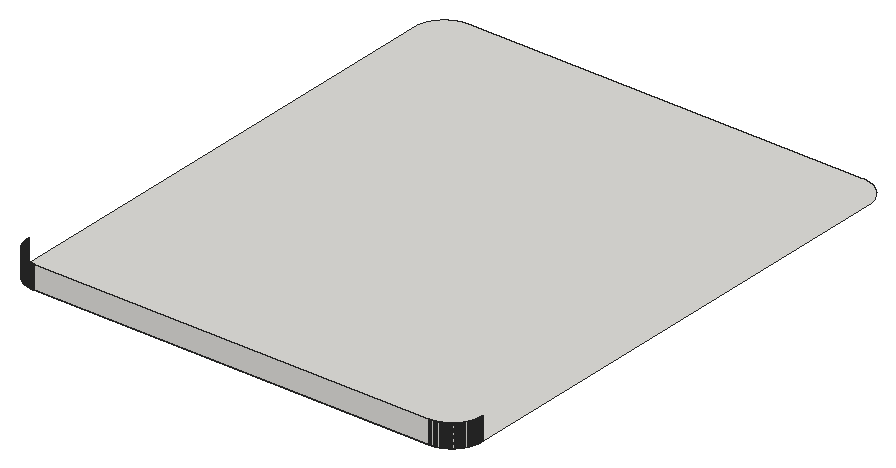
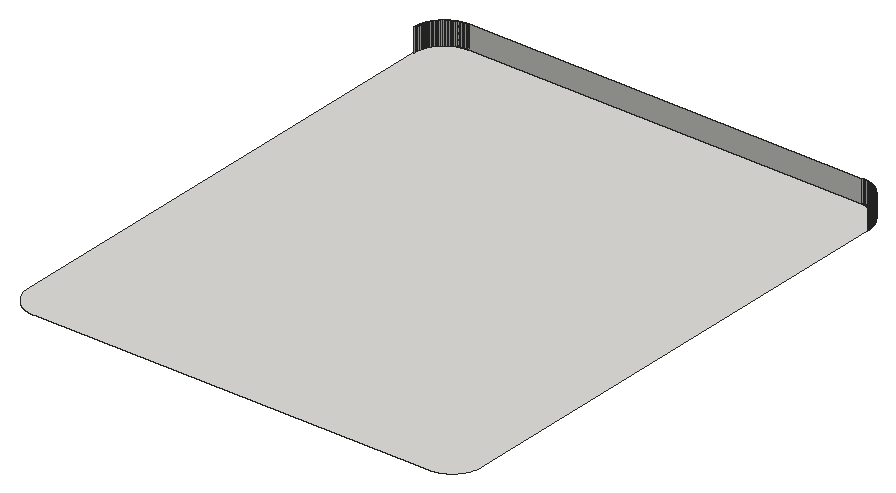
# SketchUp Ruby script. Lengths in inches.
U = 1.inch
M = Sketchup.active_model
def pt(a) = Geom::Point3d.new(a.map { |v| v * U })
def face(e, loops, mat)
  f = e.add_face(loops[0].map { |a| pt(a) })
  loops[1..].each { |l| e.add_face(l.map { |a| pt(a) }).erase! }
  f.material = f.back_material = mat if mat
  f
end
# faces: each face lists its corners as indices into pts; further lists are holes
def faces(e, pts, list, mat = nil) = list.each { |f| face(e, (f[0].is_a?(Array) ? f : [f]).map { |l| l.map { |i| pts[i] } }, mat) }
# xy, xz, yz: faces in a plane at the given z, y or x. An outline is a flat list of corners, or four numbers for a rectangle; further outlines are holes
def ring(l) = l.size == 4 ? [[l[0], l[1]], [l[2], l[1]], [l[2], l[3]], [l[0], l[3]]] : l.each_slice(2).to_a
def flat(e, list, mat, &to3) = list.each { |f| face(e, (f[0].is_a?(Array) ? f : [f]).map { |l| ring(l).map { |u, v| to3.(u, v) } }, mat) }
def xy(e, z, list, mat = nil) = flat(e, list, mat) { |x, y| [x, y, z] }
def xz(e, y, list, mat = nil) = flat(e, list, mat) { |x, z| [x, y, z] }
def yz(e, x, list, mat = nil) = flat(e, list, mat) { |y, z| [x, y, z] }
def lines(e, pts, list) = list.each { |a, b| e.add_line(pt(pts[a]), pt(pts[b])) }
# prism: a flat outline (further loops are holes) pulled along v
def prism(e, loops, v, mat = nil)
  f = face(e, loops, mat); d = Geom::Vector3d.new(v.map { |x| x * U })
  f.pushpull(f.normal.samedirection?(d) ? d.length : -d.length)
end
def box(e, o, s, mat = nil) = prism(e, [[o, [o[0] + s[0], o[1], o[2]], [o[0] + s[0], o[1] + s[1], o[2]], [o[0], o[1] + s[1], o[2]]]], [0, 0, s[2]], mat)
def at(x, y, z, deg = 0) = Geom::Transformation.translation(pt([x, y, z])) * Geom::Transformation.rotation(ORIGIN, Z_AXIS, deg.degrees)
def axes(o, x, y, z) = Geom::Transformation.new([*x, 0, *y, 0, *z, 0, *pt(o).to_a, 1])
def part(name) = M.definitions.add(name)
# library, detail: a bought-in or finely detailed component or shape, given as its bounding box
def library(name, o, s) = part(name).tap { |d| box(d.entities, o, s) }
def detail(e, o, s) = box(e.add_group.entities, o, s)
def put(e, d, t, mat = nil) = e.add_instance(d, t).tap { |i| i.material = mat if mat }
def group(e, t, mat = nil) = e.add_group.tap { |g| g.transformation = t; g.material = mat if mat }.entities
root = M.entities
M.materials.add("[Formica Graystone]").color = [224, 223, 219]
xy(root,383.82,[[17.6875,229,17.53,229.01,17.37,229.02,17.22,229.03,16.9,229.05,16.75,229.07,16.59,229.08,16.43,229.1,16.28,229.125,16.12,229.15,15.97,229.17,15.8125,229.2,15.66,229.23,15.51,229.26,15.35,229.3,15.2,229.33,15.05,229.37,14.89,229.41,14.59,229.49,14.14,229.64,13.99,229.6875,13.85,229.74,13.7,229.8,13.55,229.85,13.41,229.91,13.26,229.97,13.12,230.04,12.98,230.1,12.83,230.17,12.27,230.45,12.14,230.53,12,230.61,11.86,230.6875,11.73,230.77,11.6,230.85,11.46,230.9375,11.33,231.02,11.07,231.2,10.95,231.29,10.82,231.38,10.69,231.48,10.57,231.58,10.45,231.67,10.33,231.77,10.09,231.98,9.97,232.08,9.85,232.1875,9.74,232.3,9.625,232.4,9.51,232.51,9.4,232.625,9.3,232.74,9.1875,232.85,9.08,232.97,8.98,233.09,8.77,233.33,8.67,233.45,8.58,233.57,8.48,233.69,8.38,233.82,8.29,233.95,8.2,234.07,8.02,234.33,7.9375,234.46,7.85,234.6,7.77,234.73,7.6875,234.86,7.61,235,7.53,235.14,7.45,235.27,7.17,235.83,7.1,235.98,7.04,236.12,6.97,236.26,6.91,236.41,6.85,236.55,6.8,236.7,6.74,236.85,6.6875,236.99,6.64,237.14,6.49,237.59,6.41,237.89,6.37,238.05,6.33,238.2,6.3,238.35,6.26,238.51,6.23,238.66,6.2,238.8125,6.17,238.97,6.15,239.12,6.125,239.28,6.1,239.43,6.08,239.59,6.07,239.75,6.05,239.9,6.03,240.22,6.02,240.37,6.01,240.53,6,240.6875,6,432.3125,6.01,432.47,6.02,432.63,6.03,432.78,6.05,433.1,6.07,433.25,6.08,433.41,6.1,433.57,6.125,433.72,6.15,433.88,6.17,434.03,6.2,434.1875,6.23,434.34,6.26,434.49,6.3,434.65,6.33,434.8,6.37,434.95,6.41,435.11,6.49,435.41,6.64,435.86,6.6875,436.01,6.74,436.15,6.8,436.3,6.85,436.45,6.91,436.59,6.97,436.74,7.04,436.88,7.1,437.02,7.17,437.17,7.45,437.73,7.53,437.86,7.61,438,7.6875,438.14,7.77,438.27,7.85,438.4,7.9375,438.54,8.02,438.67,8.2,438.93,8.29,439.05,8.38,439.18,8.48,439.31,8.58,439.43,8.67,439.55,8.77,439.67,8.98,439.91,9.08,440.03,9.1875,440.15,9.3,440.26,9.4,440.375,9.51,440.49,9.625,440.6,9.74,440.7,9.85,440.8125,9.97,440.92,10.09,441.02,10.33,441.23,10.45,441.33,10.57,441.42,10.69,441.52,10.82,441.62,10.95,441.71,11.07,441.8,11.33,441.98,11.46,442.0625,11.6,442.15,11.73,442.23,11.86,442.3125,12,442.39,12.14,442.47,12.27,442.55,12.83,442.83,12.98,442.9,13.12,442.96,13.26,443.03,13.41,443.09,13.55,443.15,13.7,443.2,13.85,443.26,13.99,443.3125,14.14,443.36,14.59,443.51,14.89,443.59,15.05,443.63,15.2,443.67,15.35,443.7,15.51,443.74,15.66,443.77,15.8125,443.8,15.97,443.83,16.12,443.85,16.28,443.875,16.43,443.9,16.59,443.92,16.75,443.93,16.9,443.95,17.22,443.97,17.37,443.98,17.53,443.99,17.6875,444,174.3125,444,174.47,443.99,174.63,443.98,174.78,443.97,175.1,443.95,175.25,443.93,175.41,443.92,175.57,443.9,175.72,443.875,175.88,443.85,176.03,443.83,176.1875,443.8,176.34,443.77,176.49,443.74,176.65,443.7,176.8,443.67,176.95,443.63,177.11,443.59,177.41,443.51,177.86,443.36,178.01,443.3125,178.15,443.26,178.3,443.2,178.45,443.15,178.59,443.09,178.74,443.03,178.88,442.96,179.02,442.9,179.17,442.83,179.73,442.55,179.86,442.47,180,442.39,180.14,442.3125,180.27,442.23,180.4,442.15,180.54,442.0625,180.67,441.98,180.93,441.8,181.05,441.71,181.18,441.62,181.31,441.52,181.43,441.42,181.55,441.33,181.67,441.23,181.91,441.02,182.03,440.92,182.15,440.8125,182.26,440.7,182.375,440.6,182.49,440.49,182.6,440.375,182.7,440.26,182.8125,440.15,182.92,440.03,183.02,439.91,183.23,439.67,183.33,439.55,183.42,439.43,183.52,439.31,183.62,439.18,183.71,439.05,183.8,438.93,183.98,438.67,184.0625,438.54,184.15,438.4,184.23,438.27,184.3125,438.14,184.39,438,184.47,437.86,184.55,437.73,184.83,437.17,184.9,437.02,184.96,436.88,185.03,436.74,185.09,436.59,185.15,436.45,185.2,436.3,185.26,436.15,185.3125,436.01,185.36,435.86,185.51,435.41,185.59,435.11,185.63,434.95,185.67,434.8,185.7,434.65,185.74,434.49,185.77,434.34,185.8,434.1875,185.83,434.03,185.85,433.88,185.875,433.72,185.9,433.57,185.92,433.41,185.93,433.25,185.95,433.1,185.97,432.78,185.98,432.63,185.99,432.47,186,432.3125,186,240.6875,185.99,240.53,185.98,240.37,185.97,240.22,185.95,239.9,185.93,239.75,185.92,239.59,185.9,239.43,185.875,239.28,185.85,239.12,185.83,238.97,185.8,238.8125,185.77,238.66,185.74,238.51,185.7,238.35,185.67,238.2,185.63,238.05,185.59,237.89,185.51,237.59,185.36,237.14,185.3125,236.99,185.26,236.85,185.2,236.7,185.15,236.55,185.09,236.41,185.03,236.26,184.96,236.12,184.9,235.98,184.83,235.83,184.55,235.27,184.47,235.14,184.39,235,184.3125,234.86,184.23,234.73,184.15,234.6,184.0625,234.46,183.98,234.33,183.8,234.07,183.71,233.95,183.62,233.82,183.52,233.69,183.42,233.57,183.33,233.45,183.23,233.33,183.02,233.09,182.92,232.97,182.8125,232.85,182.7,232.74,182.6,232.625,182.49,232.51,182.375,232.4,182.26,232.3,182.15,232.1875,182.03,232.08,181.91,231.98,181.67,231.77,181.55,231.67,181.43,231.58,181.31,231.48,181.18,231.38,181.05,231.29,180.93,231.2,180.67,231.02,180.54,230.9375,180.4,230.85,180.27,230.77,180.14,230.6875,180,230.61,179.86,230.53,179.73,230.45,179.17,230.17,179.02,230.1,178.88,230.04,178.74,229.97,178.59,229.91,178.45,229.85,178.3,229.8,178.15,229.74,178.01,229.6875,177.86,229.64,177.41,229.49,177.11,229.41,176.95,229.37,176.8,229.33,176.65,229.3,176.49,229.26,176.34,229.23,176.1875,229.2,176.03,229.17,175.88,229.15,175.72,229.125,175.57,229.1,175.41,229.08,175.25,229.07,175.1,229.05,174.78,229.03,174.63,229.02,174.47,229.01,174.3125,229]],"[Formica Graystone]")
xz(root,229,[[17.6875,383.82,17.84,392.82],[17.84,383.82,18,392.82],[18,383.82,174,392.82],[174,383.82,174.16,392.82],[174.16,383.82,174.3125,392.82]],"[Formica Graystone]")
yz(root,6,[[240.6875,383.82,240.84,392.82],[240.84,383.82,241,392.82]],"[Formica Graystone]")
yz(root,186,[[240.6875,383.82,240.84,392.82],[240.84,383.82,241,392.82]],"[Formica Graystone]")
p = [[16.9,229.05,383.82],[17.06,229.04,383.82],[17.06,229.04,392.82],[16.9,229.05,392.82],[17.22,229.03,383.82],[17.22,229.03,392.82],
  [17.37,229.02,383.82],[17.37,229.02,392.82],[17.53,229.01,383.82],[17.53,229.01,392.82],[17.6875,229,383.82],[17.6875,229,392.82],
  [174.3125,229,383.82],[174.47,229.01,383.82],[174.47,229.01,392.82],[174.3125,229,392.82],[174.63,229.02,383.82],[174.63,229.02,392.82],
  [174.78,229.03,383.82],[174.78,229.03,392.82],[174.94,229.04,383.82],[174.94,229.04,392.82],[175.1,229.05,383.82],[175.1,229.05,392.82],
  [15.97,229.17,383.82],[16.12,229.15,383.82],[16.12,229.15,392.82],[15.97,229.17,392.82],[16.28,229.125,383.82],[16.28,229.125,392.82],
  [16.43,229.1,383.82],[16.43,229.1,392.82],[16.59,229.08,383.82],[16.59,229.08,392.82],[16.75,229.07,383.82],[16.75,229.07,392.82],
  [175.25,229.07,383.82],[175.25,229.07,392.82],[175.41,229.08,383.82],[175.41,229.08,392.82],[175.57,229.1,383.82],[175.57,229.1,392.82],
  [175.72,229.125,383.82],[175.72,229.125,392.82],[175.88,229.15,383.82],[175.88,229.15,392.82],[176.03,229.17,383.82],[176.03,229.17,392.82],
  [15.51,229.26,383.82],[15.66,229.23,383.82],[15.66,229.23,392.82],[15.51,229.26,392.82],[15.8125,229.2,383.82],[15.8125,229.2,392.82],
  [176.1875,229.2,383.82],[176.1875,229.2,392.82],[176.34,229.23,383.82],[176.34,229.23,392.82],[176.49,229.26,383.82],[176.49,229.26,392.82],
  [15.05,229.37,383.82],[15.2,229.33,383.82],[15.2,229.33,392.82],[15.05,229.37,392.82],[15.35,229.3,383.82],[15.35,229.3,392.82],
  [176.65,229.3,383.82],[176.65,229.3,392.82],[176.8,229.33,383.82],[176.8,229.33,392.82],[176.95,229.37,383.82],[176.95,229.37,392.82],
  [14.74,229.45,383.82],[14.89,229.41,383.82],[14.89,229.41,392.82],[14.74,229.45,392.82],[177.11,229.41,383.82],[177.11,229.41,392.82],
  [177.26,229.45,383.82],[177.26,229.45,392.82],[14.29,229.59,383.82],[14.44,229.54,383.82],[14.44,229.54,392.82],[14.29,229.59,392.82],
  [14.59,229.49,383.82],[14.59,229.49,392.82],[177.41,229.49,383.82],[177.41,229.49,392.82],[177.56,229.54,383.82],[177.56,229.54,392.82],
  [177.71,229.59,383.82],[177.71,229.59,392.82],[13.99,229.6875,383.82],[14.14,229.64,383.82],[14.14,229.64,392.82],[13.99,229.6875,392.82],
  [177.86,229.64,383.82],[177.86,229.64,392.82],[178.01,229.6875,383.82],[178.01,229.6875,392.82],[13.7,229.8,383.82],[13.85,229.74,383.82],
  [13.85,229.74,392.82],[13.7,229.8,392.82],[178.15,229.74,383.82],[178.15,229.74,392.82],[178.3,229.8,383.82],[178.3,229.8,392.82],
  [13.55,229.85,383.82],[13.55,229.85,392.82],[178.45,229.85,383.82],[178.45,229.85,392.82],[13.26,229.97,383.82],[13.41,229.91,383.82],
  [13.41,229.91,392.82],[13.26,229.97,392.82],[178.59,229.91,383.82],[178.59,229.91,392.82],[178.74,229.97,383.82],[178.74,229.97,392.82],
  [12.98,230.1,383.82],[13.12,230.04,383.82],[13.12,230.04,392.82],[12.98,230.1,392.82],[178.88,230.04,383.82],[178.88,230.04,392.82],
  [179.02,230.1,383.82],[179.02,230.1,392.82],[12.83,230.17,383.82],[12.83,230.17,392.82],[179.17,230.17,383.82],[179.17,230.17,392.82],
  [12.55,230.31,383.82],[12.69,230.24,383.82],[12.69,230.24,392.82],[12.55,230.31,392.82],[179.31,230.24,383.82],[179.31,230.24,392.82],
  [179.45,230.31,383.82],[179.45,230.31,392.82],[12.41,230.38,383.82],[12.41,230.38,392.82],[179.59,230.38,383.82],[179.59,230.38,392.82],
  [12.27,230.45,383.82],[12.27,230.45,392.82],[179.73,230.45,383.82],[179.73,230.45,392.82],[12,230.61,383.82],[12.14,230.53,383.82],
  [12.14,230.53,392.82],[12,230.61,392.82],[179.86,230.53,383.82],[179.86,230.53,392.82],[180,230.61,383.82],[180,230.61,392.82],
  [11.86,230.6875,383.82],[11.86,230.6875,392.82],[180.14,230.6875,383.82],[180.14,230.6875,392.82],[11.73,230.77,383.82],[11.73,230.77,392.82],
  [180.27,230.77,383.82],[180.27,230.77,392.82],[11.6,230.85,383.82],[11.6,230.85,392.82],[180.4,230.85,383.82],[180.4,230.85,392.82],
  [11.33,231.02,383.82],[11.46,230.9375,383.82],[11.46,230.9375,392.82],[11.33,231.02,392.82],[180.54,230.9375,383.82],[180.54,230.9375,392.82],
  [180.67,231.02,383.82],[180.67,231.02,392.82],[11.2,231.11,383.82],[11.2,231.11,392.82],[180.8,231.11,383.82],[180.8,231.11,392.82],
  [11.07,231.2,383.82],[11.07,231.2,392.82],[180.93,231.2,383.82],[180.93,231.2,392.82],[10.95,231.29,383.82],[10.95,231.29,392.82],
  [181.05,231.29,383.82],[181.05,231.29,392.82],[10.82,231.38,383.82],[10.82,231.38,392.82],[181.18,231.38,383.82],[181.18,231.38,392.82],
  [10.69,231.48,383.82],[10.69,231.48,392.82],[181.31,231.48,383.82],[181.31,231.48,392.82],[10.57,231.58,383.82],[10.57,231.58,392.82],
  [181.43,231.58,383.82],[181.43,231.58,392.82],[10.45,231.67,383.82],[10.45,231.67,392.82],[181.55,231.67,383.82],[181.55,231.67,392.82],
  [10.33,231.77,383.82],[10.33,231.77,392.82],[181.67,231.77,383.82],[181.67,231.77,392.82],[10.21,231.875,383.82],[10.21,231.875,392.82],
  [181.79,231.875,383.82],[181.79,231.875,392.82],[10.09,231.98,383.82],[10.09,231.98,392.82],[181.91,231.98,383.82],[181.91,231.98,392.82],
  [9.97,232.08,383.82],[9.97,232.08,392.82],[182.03,232.08,383.82],[182.03,232.08,392.82],[9.85,232.1875,383.82],[9.85,232.1875,392.82],
  [182.15,232.1875,383.82],[182.15,232.1875,392.82],[9.74,232.3,383.82],[9.74,232.3,392.82],[182.26,232.3,383.82],[182.26,232.3,392.82],
  [9.625,232.4,383.82],[9.625,232.4,392.82],[182.375,232.4,383.82],[182.375,232.4,392.82],[9.51,232.51,383.82],[9.51,232.51,392.82],
  [182.49,232.51,383.82],[182.49,232.51,392.82],[9.4,232.625,383.82],[9.4,232.625,392.82],[182.6,232.625,383.82],[182.6,232.625,392.82],
  [9.3,232.74,383.82],[9.3,232.74,392.82],[182.7,232.74,383.82],[182.7,232.74,392.82],[9.1875,232.85,383.82],[9.1875,232.85,392.82],
  [182.8125,232.85,383.82],[182.8125,232.85,392.82],[9.08,232.97,383.82],[9.08,232.97,392.82],[182.92,232.97,383.82],[182.92,232.97,392.82],
  [8.98,233.09,383.82],[8.98,233.09,392.82],[183.02,233.09,383.82],[183.02,233.09,392.82],[8.875,233.21,383.82],[8.875,233.21,392.82],
  [183.125,233.21,383.82],[183.125,233.21,392.82],[8.77,233.33,383.82],[8.77,233.33,392.82],[183.23,233.33,383.82],[183.23,233.33,392.82],
  [8.67,233.45,383.82],[8.67,233.45,392.82],[183.33,233.45,383.82],[183.33,233.45,392.82],[8.58,233.57,383.82],[8.58,233.57,392.82],
  [183.42,233.57,383.82],[183.42,233.57,392.82],[8.48,233.69,383.82],[8.48,233.69,392.82],[183.52,233.69,383.82],[183.52,233.69,392.82],
  [8.38,233.82,383.82],[8.38,233.82,392.82],[183.62,233.82,383.82],[183.62,233.82,392.82],[8.29,233.95,383.82],[8.29,233.95,392.82],
  [183.71,233.95,383.82],[183.71,233.95,392.82],[8.2,234.07,383.82],[8.2,234.07,392.82],[183.8,234.07,383.82],[183.8,234.07,392.82],
  [8.11,234.2,383.82],[8.11,234.2,392.82],[183.89,234.2,383.82],[183.89,234.2,392.82],[8.02,234.33,383.82],[8.02,234.33,392.82],
  [183.98,234.33,383.82],[183.98,234.33,392.82],[7.9375,234.46,383.82],[7.9375,234.46,392.82],[184.0625,234.46,383.82],[184.0625,234.46,392.82],
  [7.85,234.6,383.82],[7.85,234.6,392.82],[184.15,234.6,383.82],[184.15,234.6,392.82],[7.77,234.73,383.82],[7.77,234.73,392.82],
  [184.23,234.73,383.82],[184.23,234.73,392.82],[7.6875,234.86,383.82],[7.6875,234.86,392.82],[184.3125,234.86,383.82],[184.3125,234.86,392.82],
  [7.61,235,383.82],[7.61,235,392.82],[184.39,235,383.82],[184.39,235,392.82],[7.53,235.14,383.82],[7.53,235.14,392.82],
  [184.47,235.14,383.82],[184.47,235.14,392.82],[7.45,235.27,383.82],[7.45,235.27,392.82],[184.55,235.27,383.82],[184.55,235.27,392.82],
  [7.38,235.41,383.82],[7.38,235.41,392.82],[184.62,235.41,383.82],[184.62,235.41,392.82],[7.31,235.55,383.82],[7.31,235.55,392.82],
  [184.69,235.55,383.82],[184.69,235.55,392.82],[7.24,235.69,383.82],[7.24,235.69,392.82],[184.76,235.69,383.82],[184.76,235.69,392.82],
  [7.17,235.83,383.82],[7.17,235.83,392.82],[184.83,235.83,383.82],[184.83,235.83,392.82],[7.1,235.98,383.82],[7.1,235.98,392.82],
  [184.9,235.98,383.82],[184.9,235.98,392.82],[7.04,236.12,383.82],[7.04,236.12,392.82],[184.96,236.12,383.82],[184.96,236.12,392.82],
  [6.97,236.26,383.82],[6.97,236.26,392.82],[185.03,236.26,383.82],[185.03,236.26,392.82],[6.91,236.41,383.82],[6.91,236.41,392.82],
  [185.09,236.41,383.82],[185.09,236.41,392.82],[6.85,236.55,383.82],[6.85,236.55,392.82],[185.15,236.55,383.82],[185.15,236.55,392.82],
  [6.8,236.7,383.82],[6.8,236.7,392.82],[185.2,236.7,383.82],[185.2,236.7,392.82],[6.74,236.85,383.82],[6.74,236.85,392.82],
  [185.26,236.85,383.82],[185.26,236.85,392.82],[6.6875,236.99,383.82],[6.6875,236.99,392.82],[185.3125,236.99,383.82],[185.3125,236.99,392.82],
  [6.64,237.14,383.82],[6.64,237.14,392.82],[185.36,237.14,383.82],[185.36,237.14,392.82],[6.59,237.29,383.82],[6.59,237.29,392.82],
  [185.41,237.29,383.82],[185.41,237.29,392.82],[6.54,237.44,383.82],[6.54,237.44,392.82],[185.46,237.44,383.82],[185.46,237.44,392.82],
  [6.49,237.59,383.82],[6.49,237.59,392.82],[185.51,237.59,383.82],[185.51,237.59,392.82],[6.45,237.74,383.82],[6.45,237.74,392.82],
  [185.55,237.74,383.82],[185.55,237.74,392.82],[6.41,237.89,383.82],[6.41,237.89,392.82],[185.59,237.89,383.82],[185.59,237.89,392.82],
  [6.37,238.05,383.82],[6.37,238.05,392.82],[185.63,238.05,383.82],[185.63,238.05,392.82],[6.33,238.2,383.82],[6.33,238.2,392.82],
  [185.67,238.2,383.82],[185.67,238.2,392.82],[6.3,238.35,383.82],[6.3,238.35,392.82],[185.7,238.35,383.82],[185.7,238.35,392.82],
  [6.26,238.51,383.82],[6.26,238.51,392.82],[185.74,238.51,383.82],[185.74,238.51,392.82],[6.23,238.66,383.82],[6.23,238.66,392.82],
  [185.77,238.66,383.82],[185.77,238.66,392.82],[6.2,238.8125,383.82],[6.2,238.8125,392.82],[185.8,238.8125,383.82],[185.8,238.8125,392.82],
  [6.17,238.97,383.82],[6.17,238.97,392.82],[185.83,238.97,383.82],[185.83,238.97,392.82],[6.15,239.12,383.82],[6.15,239.12,392.82],
  [185.85,239.12,383.82],[185.85,239.12,392.82],[6.125,239.28,383.82],[6.125,239.28,392.82],[185.875,239.28,383.82],[185.875,239.28,392.82],
  [6.1,239.43,383.82],[6.1,239.43,392.82],[185.9,239.43,383.82],[185.9,239.43,392.82],[6.08,239.59,383.82],[6.08,239.59,392.82],
  [185.92,239.59,383.82],[185.92,239.59,392.82],[6.07,239.75,383.82],[6.07,239.75,392.82],[185.93,239.75,383.82],[185.93,239.75,392.82],
  [6.05,239.9,383.82],[6.05,239.9,392.82],[185.95,239.9,383.82],[185.95,239.9,392.82],[6.04,240.06,383.82],[6.04,240.06,392.82],
  [185.96,240.06,383.82],[185.96,240.06,392.82],[6.03,240.22,383.82],[6.03,240.22,392.82],[185.97,240.22,383.82],[185.97,240.22,392.82],
  [6.02,240.37,383.82],[6.02,240.37,392.82],[185.98,240.37,383.82],[185.98,240.37,392.82],[6.01,240.53,383.82],[6.01,240.53,392.82],
  [185.99,240.53,383.82],[185.99,240.53,392.82],[6,240.6875,383.82],[6,240.6875,392.82],[186,240.6875,383.82],[186,240.6875,392.82]]
faces(root,p,[[0,1,2,3],[1,4,5,2],[4,6,7,5],[6,8,9,7],[8,10,11,9],[12,13,14,15],[13,16,17,14],[16,18,19,17],
  [18,20,21,19],[20,22,23,21],[24,25,26,27],[25,28,29,26],[28,30,31,29],[30,32,33,31],[32,34,35,33],[34,0,3,35],
  [22,36,37,23],[36,38,39,37],[38,40,41,39],[40,42,43,41],[42,44,45,43],[44,46,47,45],[48,49,50,51],[49,52,53,50],
  [52,24,27,53],[46,54,55,47],[54,56,57,55],[56,58,59,57],[60,61,62,63],[61,64,65,62],[64,48,51,65],[58,66,67,59],
  [66,68,69,67],[68,70,71,69],[72,73,74,75],[73,60,63,74],[70,76,77,71],[76,78,79,77],[80,81,82,83],[81,84,85,82],
  [84,72,75,85],[78,86,87,79],[86,88,89,87],[88,90,91,89],[92,93,94,95],[93,80,83,94],[90,96,97,91],[96,98,99,97],
  [100,101,102,103],[101,92,95,102],[98,104,105,99],[104,106,107,105],[108,100,103,109],[106,110,111,107],[112,113,114,115],[113,108,109,114],
  [110,116,117,111],[116,118,119,117],[120,121,122,123],[121,112,115,122],[118,124,125,119],[124,126,127,125],[128,120,123,129],[126,130,131,127],
  [132,133,134,135],[133,128,129,134],[130,136,137,131],[136,138,139,137],[140,132,135,141],[138,142,143,139],[144,140,141,145],[142,146,147,143],
  [148,149,150,151],[149,144,145,150],[146,152,153,147],[152,154,155,153],[156,148,151,157],[154,158,159,155],[160,156,157,161],[158,162,163,159],
  [164,160,161,165],[162,166,167,163],[168,169,170,171],[169,164,165,170],[166,172,173,167],[172,174,175,173],[176,168,171,177],[174,178,179,175],
  [180,176,177,181],[178,182,183,179],[184,180,181,185],[182,186,187,183],[188,184,185,189],[186,190,191,187],[192,188,189,193],[190,194,195,191],
  [196,192,193,197],[194,198,199,195],[200,196,197,201],[198,202,203,199],[204,200,201,205],[202,206,207,203],[208,204,205,209],[206,210,211,207],
  [212,208,209,213],[210,214,215,211],[216,212,213,217],[214,218,219,215],[220,216,217,221],[218,222,223,219],[224,220,221,225],[222,226,227,223],
  [228,224,225,229],[226,230,231,227],[232,228,229,233],[230,234,235,231],[236,232,233,237],[234,238,239,235],[240,236,237,241],[238,242,243,239],
  [244,240,241,245],[242,246,247,243],[248,244,245,249],[246,250,251,247],[252,248,249,253],[250,254,255,251],[256,252,253,257],[254,258,259,255],
  [260,256,257,261],[258,262,263,259],[264,260,261,265],[262,266,267,263],[268,264,265,269],[266,270,271,267],[272,268,269,273],[270,274,275,271],
  [276,272,273,277],[274,278,279,275],[280,276,277,281],[278,282,283,279],[284,280,281,285],[282,286,287,283],[288,284,285,289],[286,290,291,287],
  [292,288,289,293],[290,294,295,291],[296,292,293,297],[294,298,299,295],[300,296,297,301],[298,302,303,299],[304,300,301,305],[302,306,307,303],
  [308,304,305,309],[306,310,311,307],[312,308,309,313],[310,314,315,311],[316,312,313,317],[314,318,319,315],[320,316,317,321],[318,322,323,319],
  [324,320,321,325],[322,326,327,323],[328,324,325,329],[326,330,331,327],[332,328,329,333],[330,334,335,331],[336,332,333,337],[334,338,339,335],
  [340,336,337,341],[338,342,343,339],[344,340,341,345],[342,346,347,343],[348,344,345,349],[346,350,351,347],[352,348,349,353],[350,354,355,351],
  [356,352,353,357],[354,358,359,355],[360,356,357,361],[358,362,363,359],[364,360,361,365],[362,366,367,363],[368,364,365,369],[366,370,371,367],
  [372,368,369,373],[370,374,375,371],[376,372,373,377],[374,378,379,375],[380,376,377,381],[378,382,383,379],[384,380,381,385],[382,386,387,383],
  [388,384,385,389],[386,390,391,387],[392,388,389,393],[390,394,395,391],[396,392,393,397],[394,398,399,395],[400,396,397,401],[398,402,403,399],
  [404,400,401,405],[402,406,407,403],[408,404,405,409],[406,410,411,407],[412,408,409,413],[410,414,415,411],[416,412,413,417],[414,418,419,415],
  [420,416,417,421],[418,422,423,419],[424,420,421,425],[422,426,427,423],[428,424,425,429],[426,430,431,427],[432,428,429,433],[430,434,435,431],
  [436,432,433,437],[434,438,439,435],[440,436,437,441],[438,442,443,439],[444,440,441,445],[442,446,447,443],[448,444,445,449],[446,450,451,447],
  [452,448,449,453],[450,454,455,451],[456,452,453,457],[454,458,459,455],[460,456,457,461],[458,462,463,459],[464,460,461,465],[462,466,467,463]],"[Formica Graystone]")
